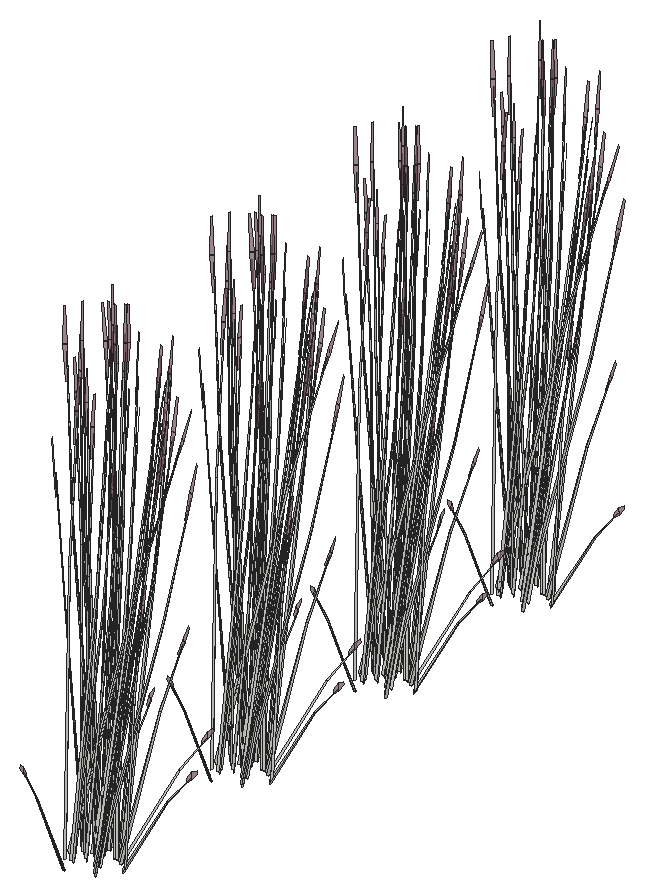
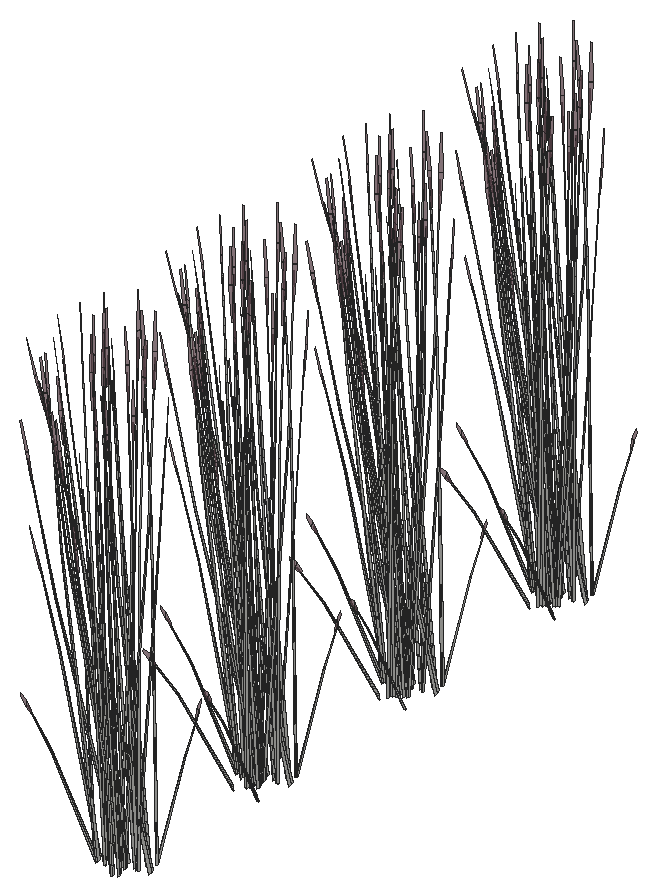
# SketchUp Ruby script. Lengths in inches.
U = 1.inch
M = Sketchup.active_model
def pt(a) = Geom::Point3d.new(a.map { |v| v * U })
def face(e, loops, mat)
  f = e.add_face(loops[0].map { |a| pt(a) })
  loops[1..].each { |l| e.add_face(l.map { |a| pt(a) }).erase! }
  f.material = f.back_material = mat if mat
  f
end
# faces: each face lists its corners as indices into pts; further lists are holes
def faces(e, pts, list, mat = nil) = list.each { |f| face(e, (f[0].is_a?(Array) ? f : [f]).map { |l| l.map { |i| pts[i] } }, mat) }
# xy, xz, yz: faces in a plane at the given z, y or x. An outline is a flat list of corners, or four numbers for a rectangle; further outlines are holes
def ring(l) = l.size == 4 ? [[l[0], l[1]], [l[2], l[1]], [l[2], l[3]], [l[0], l[3]]] : l.each_slice(2).to_a
def flat(e, list, mat, &to3) = list.each { |f| face(e, (f[0].is_a?(Array) ? f : [f]).map { |l| ring(l).map { |u, v| to3.(u, v) } }, mat) }
def xy(e, z, list, mat = nil) = flat(e, list, mat) { |x, y| [x, y, z] }
def xz(e, y, list, mat = nil) = flat(e, list, mat) { |x, z| [x, y, z] }
def yz(e, x, list, mat = nil) = flat(e, list, mat) { |y, z| [x, y, z] }
def lines(e, pts, list) = list.each { |a, b| e.add_line(pt(pts[a]), pt(pts[b])) }
# prism: a flat outline (further loops are holes) pulled along v
def prism(e, loops, v, mat = nil)
  f = face(e, loops, mat); d = Geom::Vector3d.new(v.map { |x| x * U })
  f.pushpull(f.normal.samedirection?(d) ? d.length : -d.length)
end
def box(e, o, s, mat = nil) = prism(e, [[o, [o[0] + s[0], o[1], o[2]], [o[0] + s[0], o[1] + s[1], o[2]], [o[0], o[1] + s[1], o[2]]]], [0, 0, s[2]], mat)
def at(x, y, z, deg = 0) = Geom::Transformation.translation(pt([x, y, z])) * Geom::Transformation.rotation(ORIGIN, Z_AXIS, deg.degrees)
def axes(o, x, y, z) = Geom::Transformation.new([*x, 0, *y, 0, *z, 0, *pt(o).to_a, 1])
def part(name) = M.definitions.add(name)
# library, detail: a bought-in or finely detailed component or shape, given as its bounding box
def library(name, o, s) = part(name).tap { |d| box(d.entities, o, s) }
def detail(e, o, s) = box(e.add_group.entities, o, s)
def put(e, d, t, mat = nil) = e.add_instance(d, t).tap { |i| i.material = mat if mat }
def group(e, t, mat = nil) = e.add_group.tap { |g| g.transformation = t; g.material = mat if mat }.entities
root = M.entities
M.materials.add("LightPink_Translucent").color = [144, 107, 117]
M.materials["LightPink_Translucent"].alpha = 0.75
c1 = part("blade")
p = [[2.15,0.21,22],[0,0.17,0],[0.09,0.45,0],[2.18,0.31,22],[2.29,0.31,22],[0.38,0.45,0],
  [2.48,0.24,33],[2.49,0.24,33],[2.48,0.22,33]]
faces(c1.entities,p,[[0,1,2,3],[4,5,2,3],[6,3,4,7],[8,0,3,6]])
c2 = part("seeds")
p = [[0.3,-0.1,1.38],[-0.01,-0.03,1.59],[-0.01,-0.03,0.03],[0.14,-0.07,-0.07],[0.29,-0.03,3],[0.15,0.01,3.11]]
faces(c2.entities,p,[[0,1,2,3],[1,0,4,5]],"LightPink_Translucent")
c3 = part("blade with seeds")
put(c3.entities,c1,at(0,0,0))
put(c3.entities,c2,axes([2.4,0.25,30.99],[1.5799,-0.05474,1.17369],[-0.12525,1.92788,0.29478],[-0.07173,-0.02425,1.56792]))
put(root,c3,axes([408.97,79.99,257.2],[-0.76598,-0.27433,0],[0.36864,-0.57001,0],[0,0,1.62707]))
put(root,c3,axes([410.75,80.68,257.375],[0.47504,0.61229,0],[-0.79476,0.34146,-0.51607],[-0.18101,0.07777,1.63711]))
put(root,c3,axes([409.1,103.52,257.2],[-0.76598,-0.27433,0],[0.36864,-0.57001,0],[0,0,1.62707]))
put(root,c3,axes([409.41,147.99,257.3],[-0.70674,-0.52593,-0.06131],[0.70717,-0.52625,0],[-0.02468,-0.01837,1.75571]))
put(root,c3,axes([410.87,104.2,257.375],[0.47504,0.61229,0],[-0.79476,0.34146,-0.51607],[-0.18101,0.07777,1.63711]))
put(root,c3,axes([408.41,144.17,256.49],[-0.12744,0.02202,1.76342],[-0.70477,-0.24781,-0.26939],[0.01183,-0.2067,0.30037]))
put(root,c3,axes([409.6875,125.58,257.3],[-0.70674,-0.52593,-0.06131],[0.70717,-0.52625,0],[-0.02468,-0.01837,1.75571]))
put(root,c3,axes([409.78,78.67,257.3],[-0.70674,-0.52593,-0.06131],[0.70717,-0.52625,0],[-0.02468,-0.01837,1.75571]))
put(root,c3,axes([407.98,147.39,257.36],[0.33034,0.68327,0.45755],[-0.94388,0.2376,0.17955],[0.01154,-0.12555,1.58856]))
put(root,c3,axes([407.83,147.3,257.21],[0.36864,-0.55059,-0.44739],[0.76598,0.26498,0.21531],[0,-0.12692,1.43643]))
put(root,c3,axes([410.07,127.21,257.33],[0.95122,0.19861,0.30756],[-0.23797,0.7099,-0.36492],[-0.15744,0.08885,1.64885]))
put(root,c3,axes([408.78,149.08,257.2],[-0.24791,-0.5268,0],[0.70791,-0.18448,0],[0,0,1.54371]))
put(root,c3,axes([408.6875,121.76,256.49],[-0.12744,0.02202,1.76342],[-0.70477,-0.24781,-0.26939],[0.01183,-0.2067,0.30037]))
put(root,c3,axes([409.91,102.2,257.3],[-0.70674,-0.52593,-0.06131],[0.70717,-0.52625,0],[-0.02468,-0.01837,1.75571]))
put(root,c3,axes([410.17,80.29,257.33],[0.95122,0.19861,0.30756],[-0.23797,0.7099,-0.36492],[-0.15744,0.08885,1.64885]))
put(root,c3,axes([408.78,74.85,256.49],[-0.12744,0.02202,1.76342],[-0.70477,-0.24781,-0.26939],[0.01183,-0.2067,0.30037]))
put(root,c3,axes([408.26,124.98,257.36],[0.33034,0.68327,0.45755],[-0.94388,0.2376,0.17955],[0.01154,-0.12555,1.58856]))
put(root,c3,axes([410.29,103.82,257.33],[0.95122,0.19861,0.30756],[-0.23797,0.7099,-0.36492],[-0.15744,0.08885,1.64885]))
put(root,c3,axes([408.91,98.375,256.49],[-0.12744,0.02202,1.76342],[-0.70477,-0.24781,-0.26939],[0.01183,-0.2067,0.30037]))
put(root,c3,axes([408.11,124.89,257.21],[0.36864,-0.55059,-0.44739],[0.76598,0.26498,0.21531],[0,-0.12692,1.43643]))
put(root,c3,axes([409.05,126.67,257.2],[-0.24791,-0.5268,0],[0.70791,-0.18448,0],[0,0,1.54371]))
put(root,c3,axes([408.36,78.0625,257.36],[0.33034,0.68327,0.45755],[-0.94388,0.2376,0.17955],[0.01154,-0.12555,1.58856]))
put(root,c3,axes([408.15,127.78,256.49],[0.12297,-0.03325,1.76342],[0.73967,0.18301,-0.26939],[0.02163,0.20626,0.30037]))
put(root,c3,axes([408.2,77.98,257.21],[0.36864,-0.55059,-0.44739],[0.76598,0.26498,0.21531],[0,-0.12692,1.43643]))
put(root,c3,axes([409.15,79.75,257.2],[-0.24791,-0.5268,0],[0.70791,-0.18448,0],[0,0,1.54371]))
put(root,c3,axes([408.25,80.86,256.49],[0.12297,-0.03325,1.76342],[0.73967,0.18301,-0.26939],[0.02163,0.20626,0.30037]))
put(root,c3,axes([408.33,101.5,257.21],[0.36864,-0.55059,-0.44739],[0.76598,0.26498,0.21531],[0,-0.12692,1.43643]))
put(root,c3,axes([409.27,103.28,257.2],[-0.24791,-0.5268,0],[0.70791,-0.18448,0],[0,0,1.54371]))
put(root,c3,axes([408.37,104.39,256.49],[0.12297,-0.03325,1.76342],[0.73967,0.18301,-0.26939],[0.02163,0.20626,0.30037]))
put(root,c3,axes([410.06,125.63,257.21],[-0.36864,0.55059,-0.44739],[-0.76598,-0.26498,0.21531],[0,0.12692,1.43643]))
put(root,c3,axes([409.17,147.44,257.21],[0,-0.70701,0],[0.95008,0,0],[0,0,1.79456]))
put(root,c3,axes([409.65,147.73,257.29],[0,0.70667,-0.05637],[-0.95008,0,0],[0,0.02221,1.79368]))
put(root,c3,axes([410.15,78.71,257.21],[-0.36864,0.55059,-0.44739],[-0.76598,-0.26498,0.21531],[0,0.12692,1.43643]))
put(root,c3,axes([410.27,102.24,257.21],[-0.36864,0.55059,-0.44739],[-0.76598,-0.26498,0.21531],[0,0.12692,1.43643]))
put(root,c3,axes([409.45,125.03,257.21],[0,-0.70701,0],[0.95008,0,0],[0,0,1.79456]))
put(root,c3,axes([409.19,149.09,257.29],[0.33034,0.70197,-0.06012],[-0.94388,0.24598,0],[0.01154,0.02451,1.72173]))
put(root,c3,axes([409.93,125.32,257.29],[0,0.70667,-0.05637],[-0.95008,0,0],[0,0.02221,1.79368]))
put(root,c3,axes([409.54,78.12,257.21],[0,-0.70701,0],[0.95008,0,0],[0,0,1.79456]))
put(root,c3,axes([410.02,78.4,257.29],[0,0.70667,-0.05637],[-0.95008,0,0],[0,0.02221,1.79368]))
put(root,c3,axes([409.67,101.65,257.21],[0,-0.70701,0],[0.95008,0,0],[0,0,1.79456]))
put(root,c3,axes([410.15,101.93,257.29],[0,0.70667,-0.05637],[-0.95008,0,0],[0,0.02221,1.79368]))
put(root,c3,axes([409.47,126.68,257.29],[0.33034,0.70197,-0.06012],[-0.94388,0.24598,0],[0.01154,0.02451,1.72173]))
put(root,c3,axes([407.23,145.34,257.375],[-0.47504,-0.61229,0],[0.79476,-0.34146,-0.51607],[0.18101,-0.07777,1.63711]))
put(root,c3,axes([411.92,148.17,257.2],[-0.94962,-0.00489,-0.04976],[0,-0.68292,0.49943],[-0.02984,0.15546,1.58352]))
put(root,c3,axes([409.57,79.77,257.29],[0.33034,0.70197,-0.06012],[-0.94388,0.24598,0],[0.01154,0.02451,1.72173]))
put(root,c3,axes([409.69,103.3,257.29],[0.33034,0.70197,-0.06012],[-0.94388,0.24598,0],[0.01154,0.02451,1.72173]))
put(root,c3,axes([407.51,122.93,257.375],[-0.47504,-0.61229,0],[0.79476,-0.34146,-0.51607],[0.18101,-0.07777,1.63711]))
put(root,c3,axes([412.2,125.76,257.2],[-0.94962,-0.00489,-0.04976],[0,-0.68292,0.49943],[-0.02984,0.15546,1.58352]))
put(root,c3,axes([407.61,76.01,257.375],[-0.47504,-0.61229,0],[0.79476,-0.34146,-0.51607],[0.18101,-0.07777,1.63711]))
put(root,c3,axes([412.29,78.85,257.2],[-0.94962,-0.00489,-0.04976],[0,-0.68292,0.49943],[-0.02984,0.15546,1.58352]))
put(root,c3,axes([408.72,147,257.36],[-0.62999,0.55453,0.45755],[-0.74845,-0.4895,0.17955],[0.15188,-0.05534,1.58856]))
put(root,c3,axes([409.8,147.875,257.21],[0.53038,0.39469,0],[-0.53038,0.39469,0],[0,0,1.69266]))
put(root,c3,axes([407.73,99.54,257.375],[-0.47504,-0.61229,0],[0.79476,-0.34146,-0.51607],[0.18101,-0.07777,1.63711]))
put(root,c3,axes([409.47,149.32,257.2],[0.76598,0.27433,0],[-0.36864,0.57001,0],[0,0,1.74954]))
put(root,c3,axes([412.42,102.38,257.2],[-0.94962,-0.00489,-0.04976],[0,-0.68292,0.49943],[-0.02984,0.15546,1.58352]))
put(root,c3,axes([409,124.59,257.36],[-0.62999,0.55453,0.45755],[-0.74845,-0.4895,0.17955],[0.15188,-0.05534,1.58856]))
put(root,c3,axes([410.08,125.46,257.21],[0.53038,0.39469,0],[-0.53038,0.39469,0],[0,0,1.69266]))
put(root,c3,axes([409.75,126.91,257.2],[0.76598,0.27433,0],[-0.36864,0.57001,0],[0,0,1.74954]))
put(root,c3,axes([409.09,77.68,257.36],[-0.62999,0.55453,0.45755],[-0.74845,-0.4895,0.17955],[0.15188,-0.05534,1.58856]))
put(root,c3,axes([410.17,78.55,257.21],[0.53038,0.39469,0],[-0.53038,0.39469,0],[0,0,1.69266]))
put(root,c3,axes([411.73,148.27,257.03],[-0.53038,0.38124,-0.30978],[-0.53038,-0.38124,0.30978],[0,0.1228,1.38974]))
put(root,c3,axes([409.84,80,257.2],[0.76598,0.27433,0],[-0.36864,0.57001,0],[0,0,1.74954]))
put(root,c3,axes([410.29,102.08,257.21],[0.53038,0.39469,0],[-0.53038,0.39469,0],[0,0,1.69266]))
put(root,c3,axes([409.97,103.53,257.2],[0.76598,0.27433,0],[-0.36864,0.57001,0],[0,0,1.74954]))
put(root,c3,axes([409.82,147.6,257.21],[0.85008,0,0],[0,0.63259,0],[0,0,1.78407]))
put(root,c3,axes([412,125.86,257.03],[-0.53038,0.38124,-0.30978],[-0.53038,-0.38124,0.30978],[0,0.1228,1.38974]))
put(root,c3,axes([408.17,147.03,257.67],[-0.08854,-0.69723,-0.29095],[0.92215,-0.04216,-0.50002],[0.16238,-0.09287,1.59708]))
put(root,c3,axes([412.1,78.95,257.03],[-0.53038,0.38124,-0.30978],[-0.53038,-0.38124,0.30978],[0,0.1228,1.38974]))
put(root,c3,axes([410.49,125.79,257.09],[0.2786,0.55945,-0.69212],[-0.80253,0.20149,-0.18165],[0.03079,0.18945,1.52773]))
put(root,c3,axes([410.1,125.19,257.21],[0.85008,0,0],[0,0.63259,0],[0,0,1.78407]))
put(root,c3,axes([412.22,102.48,257.03],[-0.53038,0.38124,-0.30978],[-0.53038,-0.38124,0.30978],[0,0.1228,1.38974]))
put(root,c3,axes([410.58,78.88,257.09],[0.2786,0.55945,-0.69212],[-0.80253,0.20149,-0.18165],[0.03079,0.18945,1.52773]))
put(root,c3,axes([410.1875,78.28,257.21],[0.85008,0,0],[0,0.63259,0],[0,0,1.78407]))
put(root,c3,axes([408.45,124.62,257.67],[-0.08854,-0.69723,-0.29095],[0.92215,-0.04216,-0.50002],[0.16238,-0.09287,1.59708]))
put(root,c3,axes([410.71,102.41,257.09],[0.2786,0.55945,-0.69212],[-0.80253,0.20149,-0.18165],[0.03079,0.18945,1.52773]))
put(root,c3,axes([409.87,147.58,257.67],[0.85568,0.29155,-0.29095],[-0.41201,0.61537,-0.50002],[0.02689,0.15109,1.59708]))
put(root,c3,axes([410.3125,101.81,257.21],[0.85008,0,0],[0,0.63259,0],[0,0,1.78407]))
put(root,c3,axes([408.54,77.7,257.67],[-0.08854,-0.69723,-0.29095],[0.92215,-0.04216,-0.50002],[0.16238,-0.09287,1.59708]))
put(root,c3,axes([408.05,145.48,257.03],[0.70886,0.15119,-0.30978],[-0.17848,0.53243,0.30978],[0.1429,-0.0614,1.38974]))
put(root,c3,axes([408.66,101.23,257.67],[-0.08854,-0.69723,-0.29095],[0.92215,-0.04216,-0.50002],[0.16238,-0.09287,1.59708]))
put(root,c3,axes([410.15,125.17,257.67],[0.85568,0.29155,-0.29095],[-0.41201,0.61537,-0.50002],[0.02689,0.15109,1.59708]))
put(root,c3,axes([410.24,78.26,257.67],[0.85568,0.29155,-0.29095],[-0.41201,0.61537,-0.50002],[0.02689,0.15109,1.59708]))
put(root,c3,axes([408.33,123.07,257.03],[0.70886,0.15119,-0.30978],[-0.17848,0.53243,0.30978],[0.1429,-0.0614,1.38974]))
put(root,c3,axes([407.88,145.24,257.02],[0.7111,-0.30552,-0.49651],[0.42504,0.54784,0],[0.16196,-0.06958,1.57504]))
put(root,c3,axes([408.42,76.16,257.03],[0.70886,0.15119,-0.30978],[-0.17848,0.53243,0.30978],[0.1429,-0.0614,1.38974]))
put(root,c3,axes([410.37,101.78,257.67],[0.85568,0.29155,-0.29095],[-0.41201,0.61537,-0.50002],[0.02689,0.15109,1.59708]))
put(root,c3,axes([408.54,99.6875,257.03],[0.70886,0.15119,-0.30978],[-0.17848,0.53243,0.30978],[0.1429,-0.0614,1.38974]))
put(root,c3,axes([412.37,125.875,257.02],[0,0.61104,-0.49651],[-0.85008,0,0],[0,0.13917,1.57504]))
put(root,c3,axes([408.16,122.83,257.02],[0.7111,-0.30552,-0.49651],[0.42504,0.54784,0],[0.16196,-0.06958,1.57504]))
put(root,c3,axes([412.46,78.96,257.02],[0,0.61104,-0.49651],[-0.85008,0,0],[0,0.13917,1.57504]))
put(root,c3,axes([408.25,75.92,257.02],[0.7111,-0.30552,-0.49651],[0.42504,0.54784,0],[0.16196,-0.06958,1.57504]))
put(root,c3,axes([412.59,102.49,257.02],[0,0.61104,-0.49651],[-0.85008,0,0],[0,0.13917,1.57504]))
put(root,c3,axes([408.375,99.45,257.02],[0.7111,-0.30552,-0.49651],[0.42504,0.54784,0],[0.16196,-0.06958,1.57504]))
put(root,c3,axes([409.7,149,257.18],[0.79769,-0.20732,-0.19198],[0.2803,0.59721,0.00008],[0.08805,-0.02292,1.73897]))
put(root,c3,axes([409.98,126.59,257.18],[0.79769,-0.20732,-0.19198],[0.2803,0.59721,0.00008],[0.08805,-0.02292,1.73897]))
put(root,c3,axes([410.08,79.68,257.18],[0.79769,-0.20732,-0.19198],[0.2803,0.59721,0.00008],[0.08805,-0.02292,1.73897]))
put(root,c3,axes([409.72,147.23,257.21],[0.45644,0.51287,-0.44739],[-0.69137,0.36116,0.21531],[0.14771,0.06346,1.43643]))
put(root,c3,axes([410.2,103.21,257.18],[0.79769,-0.20732,-0.19198],[0.2803,0.59721,0.00008],[0.08805,-0.02292,1.73897]))
put(root,c3,axes([410,124.82,257.21],[0.45644,0.51287,-0.44739],[-0.69137,0.36116,0.21531],[0.14771,0.06346,1.43643]))
put(root,c3,axes([410.09,77.9,257.21],[0.45644,0.51287,-0.44739],[-0.69137,0.36116,0.21531],[0.14771,0.06346,1.43643]))
put(root,c3,axes([408.72,146.5,257.06],[0.51177,-0.45928,-0.62353],[0.63575,0.41646,-0.16365],[0.20507,-0.11457,1.37633]))
put(root,c3,axes([410.22,101.43,257.21],[0.45644,0.51287,-0.44739],[-0.69137,0.36116,0.21531],[0.14771,0.06346,1.43643]))
put(root,c3,axes([409,124.09,257.06],[0.51177,-0.45928,-0.62353],[0.63575,0.41646,-0.16365],[0.20507,-0.11457,1.37633]))
put(root,c3,axes([410.97,146.09,257.03],[0.17848,0.53243,-0.30978],[-0.70886,0.15119,0.30978],[0.1429,0.0614,1.38974]))
put(root,c3,axes([412.3,147.82,257.375],[0.95008,0,0],[0,0.68292,-0.51607],[0,0.15554,1.63711]))
put(root,c3,axes([409.09,77.17,257.06],[0.51177,-0.45928,-0.62353],[0.63575,0.41646,-0.16365],[0.20507,-0.11457,1.37633]))
put(root,c3,axes([409.22,100.7,257.06],[0.51177,-0.45928,-0.62353],[0.63575,0.41646,-0.16365],[0.20507,-0.11457,1.37633]))
put(root,c3,axes([409.23,146.9375,257.67],[0.76714,-0.40567,-0.29095],[0.51013,0.57321,-0.50002],[0.18927,0.05821,1.59708]))
put(root,c3,axes([411.25,123.68,257.03],[0.17848,0.53243,-0.30978],[-0.70886,0.15119,0.30978],[0.1429,0.0614,1.38974]))
put(root,c3,axes([412.58,125.41,257.375],[0.95008,0,0],[0,0.68292,-0.51607],[0,0.15554,1.63711]))
put(root,c3,axes([411.34,76.77,257.03],[0.17848,0.53243,-0.30978],[-0.70886,0.15119,0.30978],[0.1429,0.0614,1.38974]))
put(root,c3,axes([412.67,78.5,257.375],[0.95008,0,0],[0,0.68292,-0.51607],[0,0.15554,1.63711]))
put(root,c3,axes([409.51,124.53,257.67],[0.76714,-0.40567,-0.29095],[0.51013,0.57321,-0.50002],[0.18927,0.05821,1.59708]))
put(root,c3,axes([411.46,100.29,257.03],[0.17848,0.53243,-0.30978],[-0.70886,0.15119,0.30978],[0.1429,0.0614,1.38974]))
put(root,c3,axes([412.8,102.03,257.375],[0.95008,0,0],[0,0.68292,-0.51607],[0,0.15554,1.63711]))
put(root,c3,axes([409.6,77.62,257.67],[0.76714,-0.40567,-0.29095],[0.51013,0.57321,-0.50002],[0.18927,0.05821,1.59708]))
put(root,c3,axes([409.73,101.14,257.67],[0.76714,-0.40567,-0.29095],[0.51013,0.57321,-0.50002],[0.18927,0.05821,1.59708]))
put(root,c3,axes([407.3,146.58,256.59],[-0.74787,0.24464,1.28929],[-0.23804,-0.70192,0.50096],[0.45924,0.01168,1.46642]))
put(root,c3,axes([407.57,124.17,256.59],[-0.74787,0.24464,1.28929],[-0.23804,-0.70192,0.50096],[0.45924,0.01168,1.46642]))
put(root,c3,axes([407.67,77.25,256.59],[-0.74787,0.24464,1.28929],[-0.23804,-0.70192,0.50096],[0.45924,0.01168,1.46642]))
put(root,c3,axes([410.73,145.49,257.375],[0.47504,-0.61229,0],[0.79476,0.34146,-0.51607],[0.18101,0.07777,1.63711]))
put(root,c3,axes([411.53,145.22,256.49],[-0.11372,-0.04814,1.76342],[-0.29211,-0.53779,-0.26939],[0.19706,-0.14594,0.30037]))
put(root,c3,axes([407.79,100.78,256.59],[-0.74787,0.24464,1.28929],[-0.23804,-0.70192,0.50096],[0.45924,0.01168,1.46642]))
put(root,c3,axes([411.17,145.86,257.02],[0.7111,0.30552,-0.49651],[-0.42504,0.54784,0],[0.16196,0.06958,1.57504]))
put(root,c3,axes([411.01,123.08,257.375],[0.47504,-0.61229,0],[0.79476,0.34146,-0.51607],[0.18101,0.07777,1.63711]))
put(root,c3,axes([411.81,122.8125,256.49],[-0.11372,-0.04814,1.76342],[-0.29211,-0.53779,-0.26939],[0.19706,-0.14594,0.30037]))
put(root,c3,axes([411.1,76.17,257.375],[0.47504,-0.61229,0],[0.79476,0.34146,-0.51607],[0.18101,0.07777,1.63711]))
put(root,c3,axes([411.9,75.9,256.49],[-0.11372,-0.04814,1.76342],[-0.29211,-0.53779,-0.26939],[0.19706,-0.14594,0.30037]))
put(root,c3,axes([411.44,123.45,257.02],[0.7111,0.30552,-0.49651],[-0.42504,0.54784,0],[0.16196,0.06958,1.57504]))
put(root,c3,axes([411.23,99.69,257.375],[0.47504,-0.61229,0],[0.79476,0.34146,-0.51607],[0.18101,0.07777,1.63711]))
put(root,c3,axes([412.03,99.43,256.49],[-0.11372,-0.04814,1.76342],[-0.29211,-0.53779,-0.26939],[0.19706,-0.14594,0.30037]))
put(root,c3,axes([411.54,76.54,257.02],[0.7111,0.30552,-0.49651],[-0.42504,0.54784,0],[0.16196,0.06958,1.57504]))
put(root,c3,axes([411.41,127.8,256.49],[0.05536,-0.08822,1.76342],[0.69692,-0.25981,-0.26939],[0.21129,0.13447,0.30037]))
put(root,c3,axes([410.13,147.03,257.06],[0.79037,0.10018,-0.62353],[-0.16679,0.61794,-0.16365],[0.23587,0.07488,1.37633]))
put(root,c3,axes([411.66,100.0625,257.02],[0.7111,0.30552,-0.49651],[-0.42504,0.54784,0],[0.16196,0.06958,1.57504]))
put(root,c3,axes([411.5,80.88,256.49],[0.05536,-0.08822,1.76342],[0.69692,-0.25981,-0.26939],[0.21129,0.13447,0.30037]))
put(root,c3,axes([413.49,147.39,257.26],[-0.47106,-0.39072,-0.06488],[0.51591,-0.35801,-0.29416],[0.14618,-0.02521,0.97024]))
put(root,c3,axes([411.63,104.41,256.49],[0.05536,-0.08822,1.76342],[0.69692,-0.25981,-0.26939],[0.21129,0.13447,0.30037]))
put(root,c3,axes([410.41,124.62,257.06],[0.79037,0.10018,-0.62353],[-0.16679,0.61794,-0.16365],[0.23587,0.07488,1.37633]))
put(root,c3,axes([413.77,124.98,257.26],[-0.47106,-0.39072,-0.06488],[0.51591,-0.35801,-0.29416],[0.14618,-0.02521,0.97024]))
put(root,c3,axes([410.5,77.71,257.06],[0.79037,0.10018,-0.62353],[-0.16679,0.61794,-0.16365],[0.23587,0.07488,1.37633]))
put(root,c3,axes([413.87,78.07,257.26],[-0.47106,-0.39072,-0.06488],[0.51591,-0.35801,-0.29416],[0.14618,-0.02521,0.97024]))
put(root,c3,axes([410.625,101.23,257.06],[0.79037,0.10018,-0.62353],[-0.16679,0.61794,-0.16365],[0.23587,0.07488,1.37633]))
put(root,c3,axes([413.99,101.6,257.26],[-0.47106,-0.39072,-0.06488],[0.51591,-0.35801,-0.29416],[0.14618,-0.02521,0.97024]))
put(root,c3,axes([412.6,147.91,256.98],[-0.48937,0.07333,1.41583],[-0.07789,-0.58369,0.08104],[0.34275,-0.08835,0.80566]))
put(root,c3,axes([413.14,147.53,256.49],[-0.03971,-0.09277,1.76342],[0.27541,-0.54264,-0.26939],[0.27782,-0.00781,0.30037]))
put(root,c3,axes([412.88,125.5,256.98],[-0.48937,0.07333,1.41583],[-0.07789,-0.58369,0.08104],[0.34275,-0.08835,0.80566]))
put(root,c3,axes([413.42,125.12,256.49],[-0.03971,-0.09277,1.76342],[0.27541,-0.54264,-0.26939],[0.27782,-0.00781,0.30037]))
put(root,c3,axes([412.97,78.59,256.98],[-0.48937,0.07333,1.41583],[-0.07789,-0.58369,0.08104],[0.34275,-0.08835,0.80566]))
put(root,c3,axes([413.51,78.21,256.49],[-0.03971,-0.09277,1.76342],[0.27541,-0.54264,-0.26939],[0.27782,-0.00781,0.30037]))
put(root,c3,axes([413.1,102.11,256.98],[-0.48937,0.07333,1.41583],[-0.07789,-0.58369,0.08104],[0.34275,-0.08835,0.80566]))
put(root,c3,axes([413.63,101.73,256.49],[-0.03971,-0.09277,1.76342],[0.27541,-0.54264,-0.26939],[0.27782,-0.00781,0.30037]))
